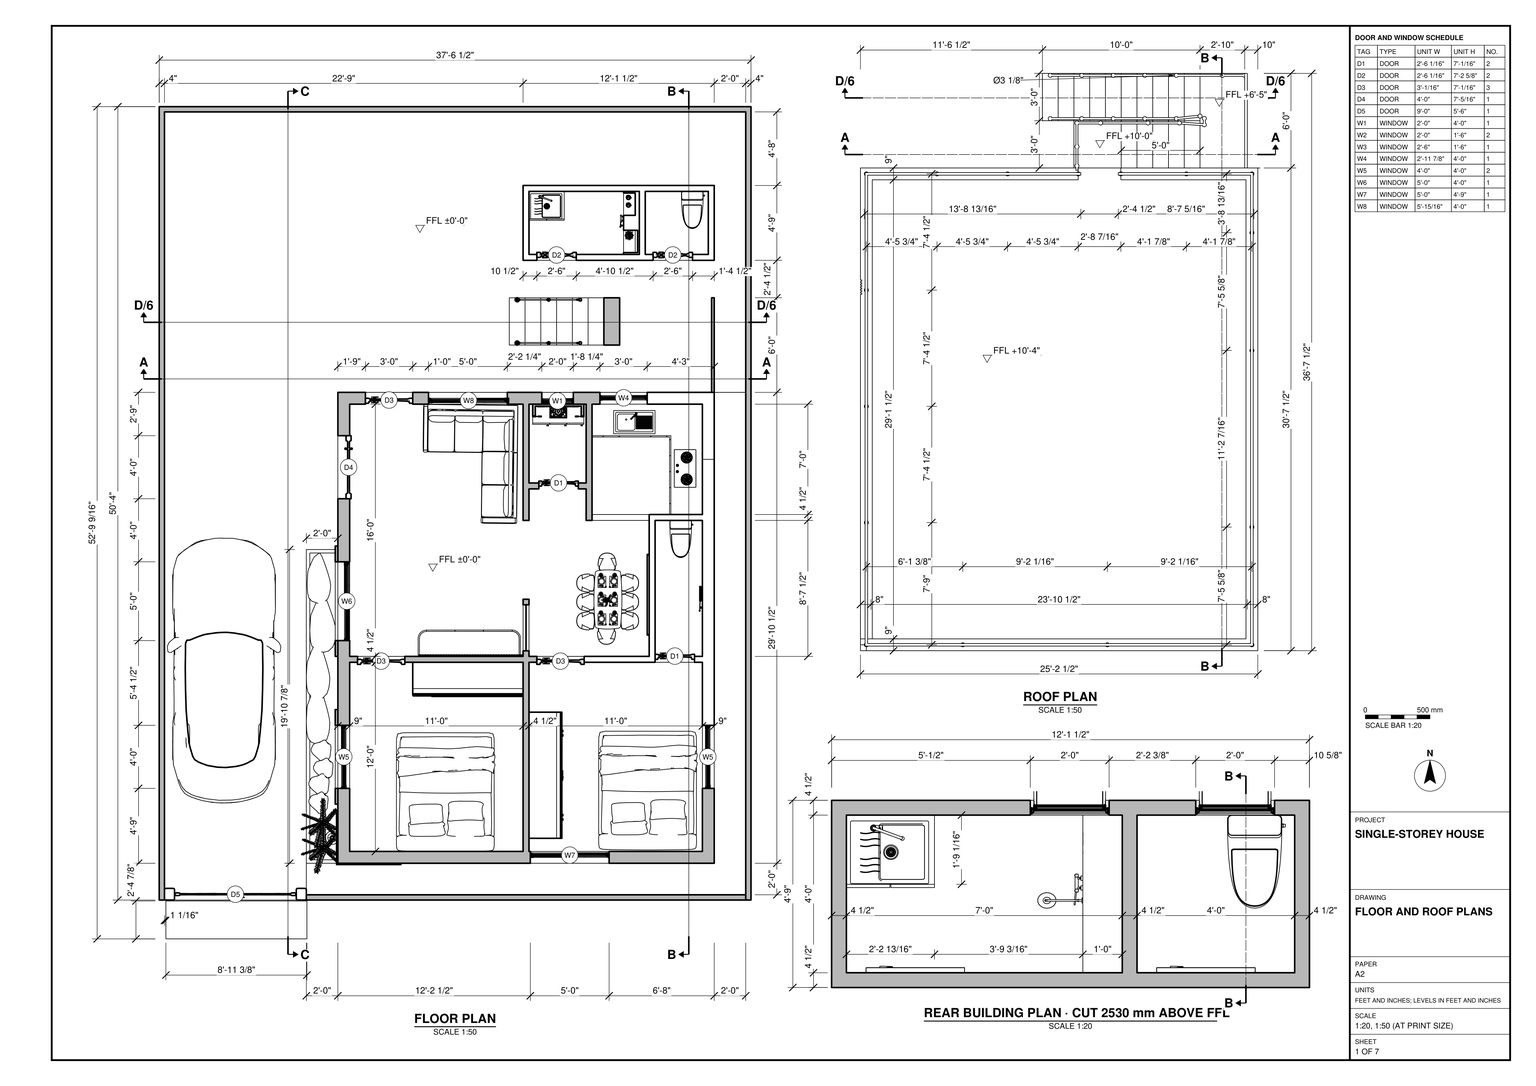
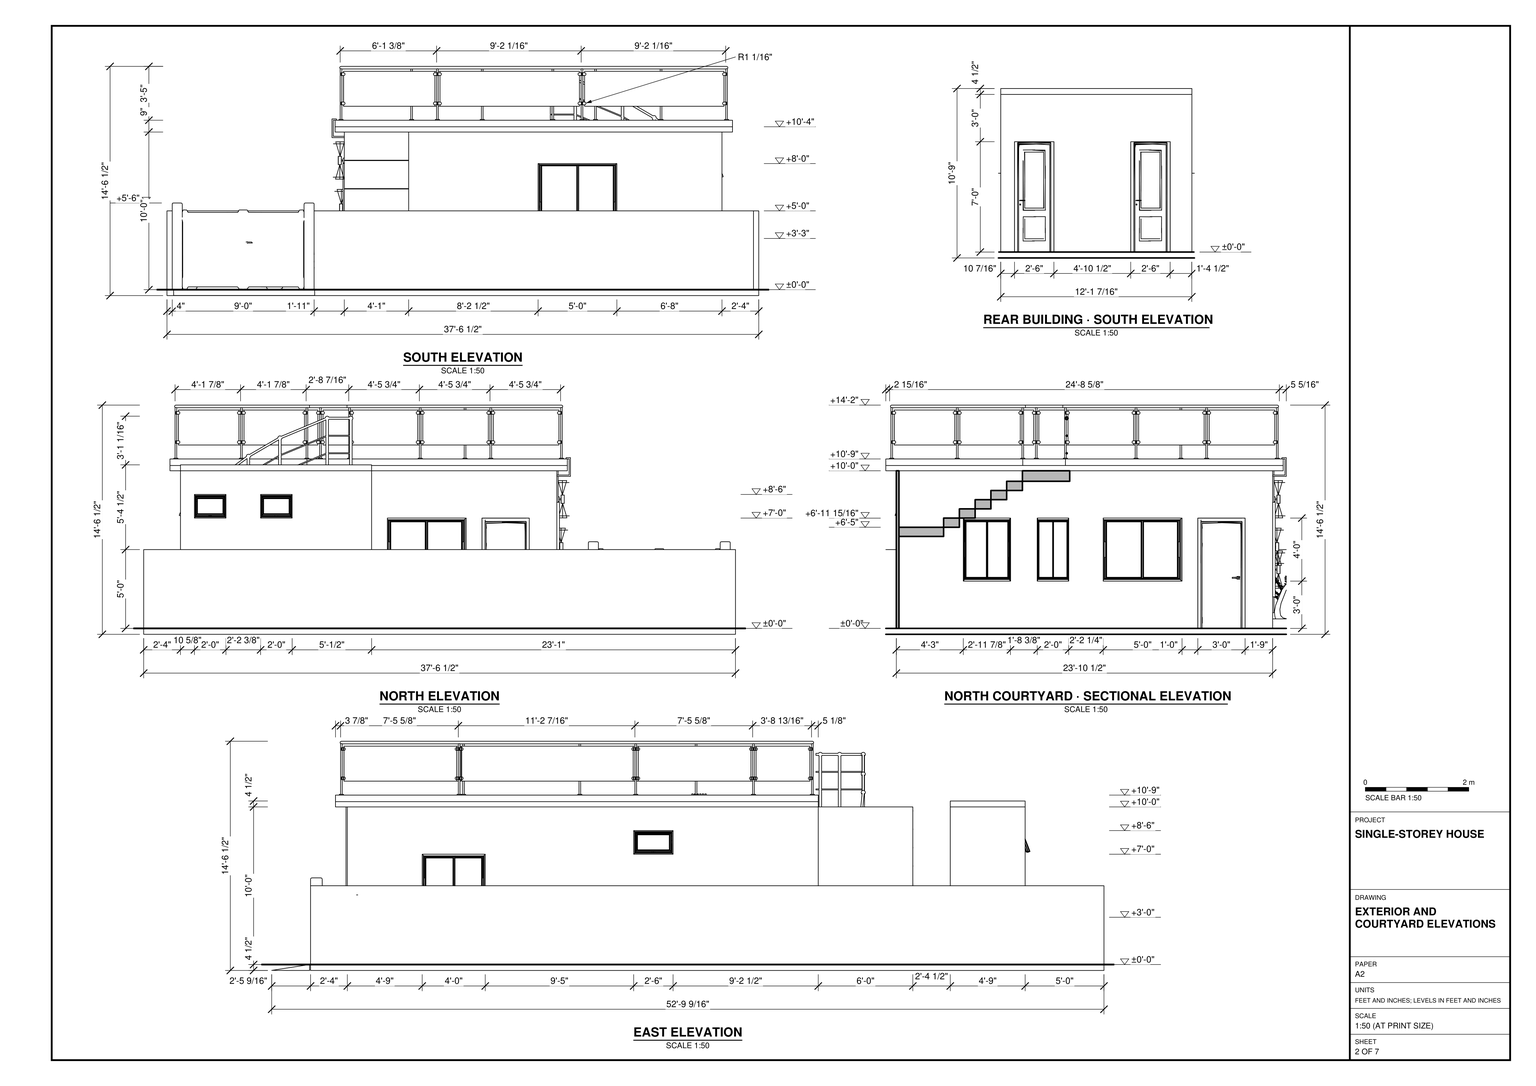
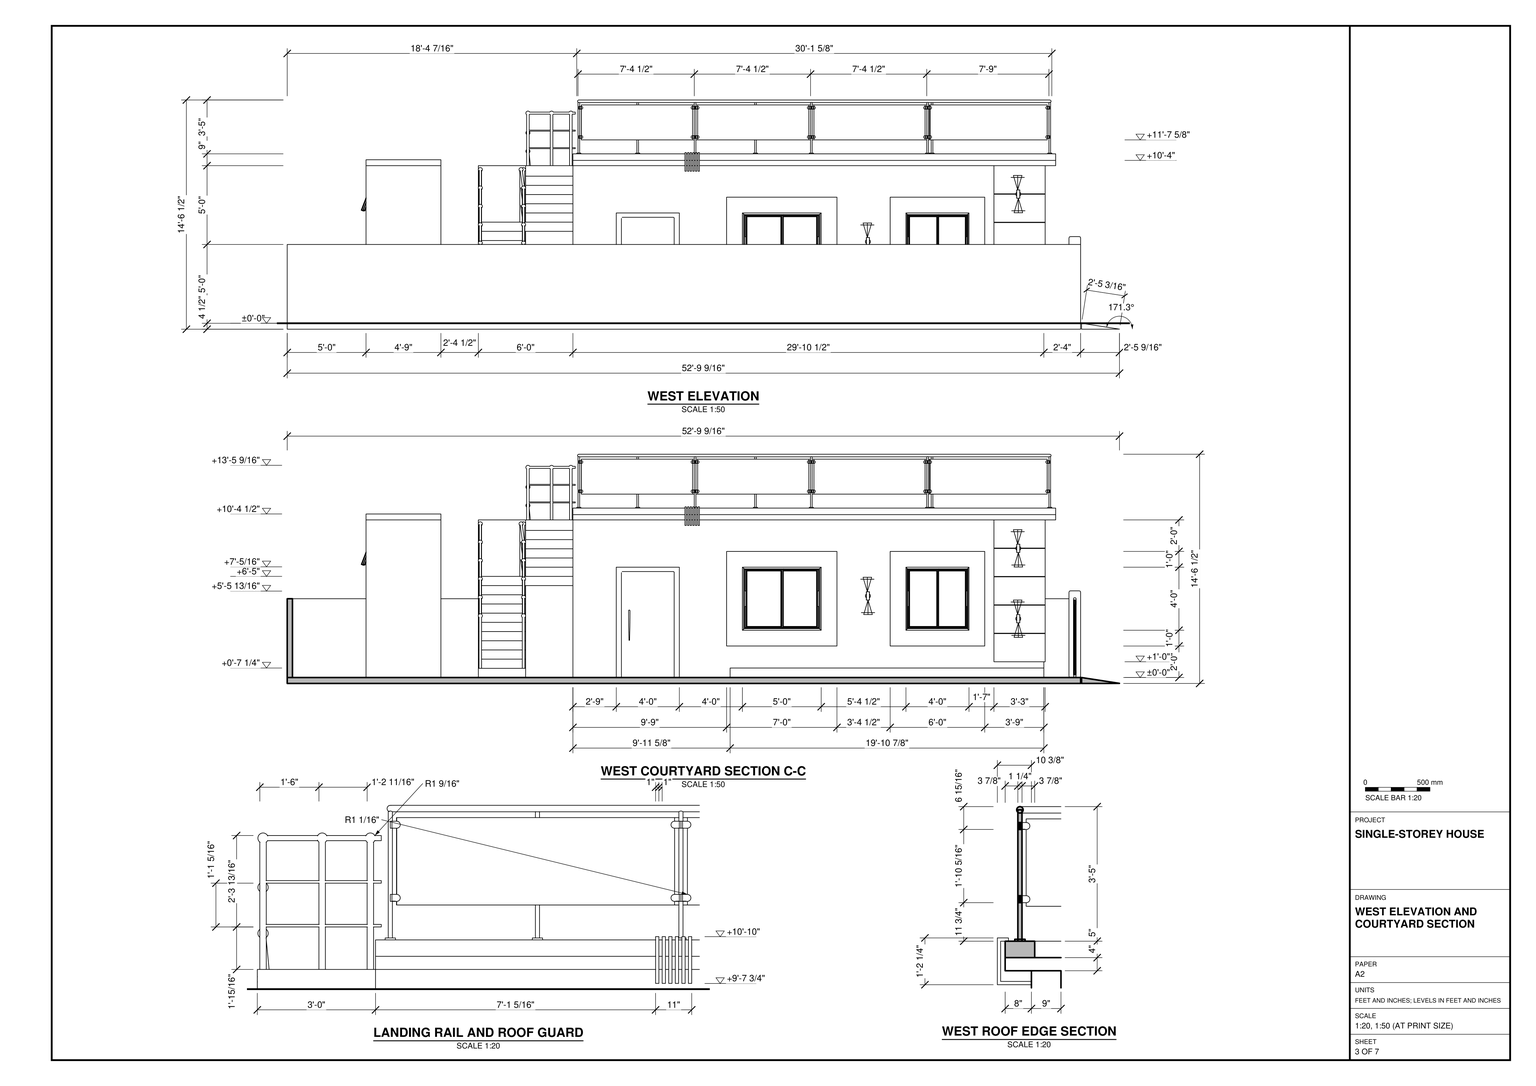
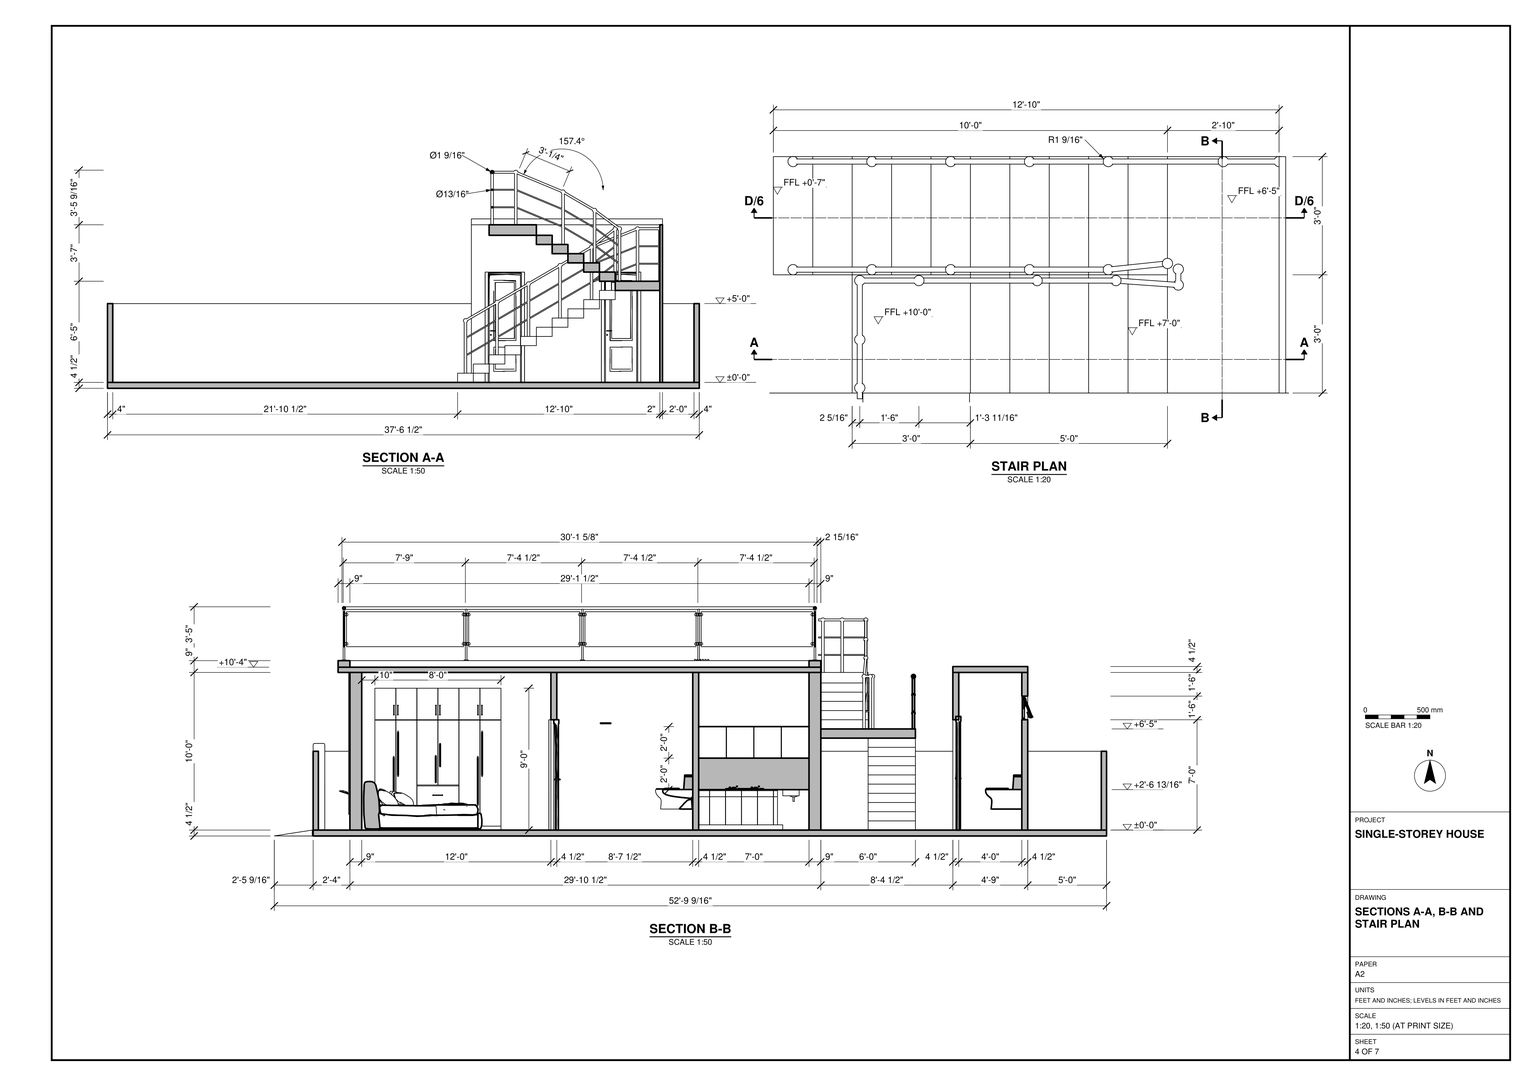
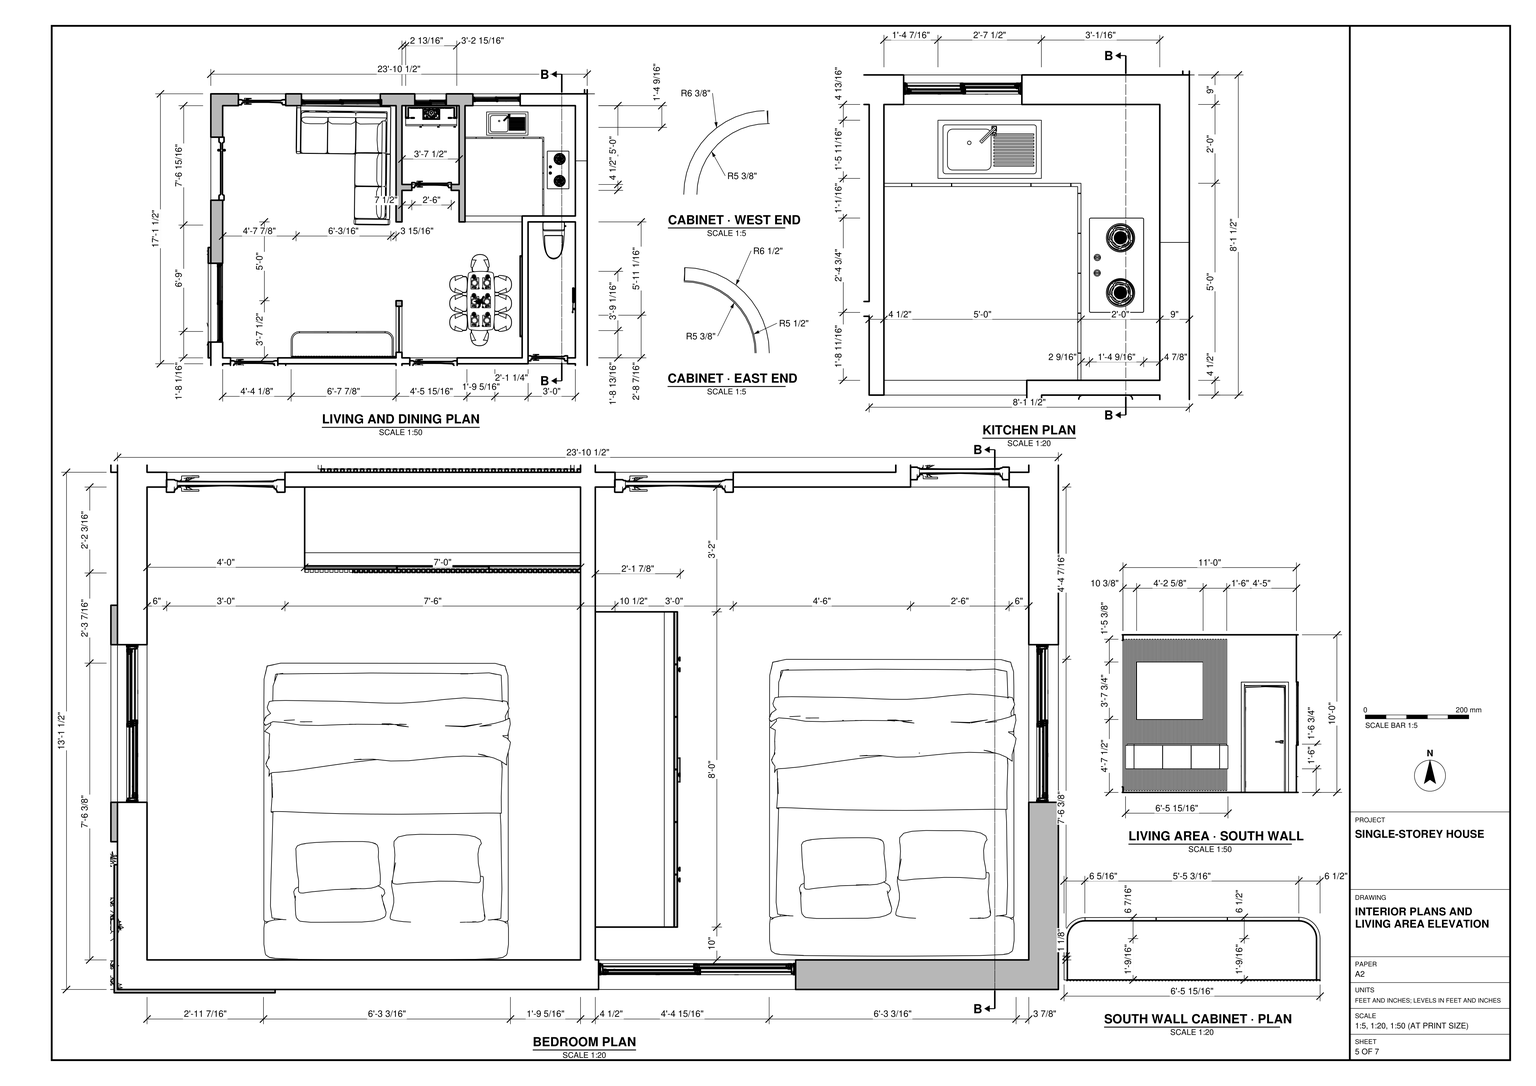
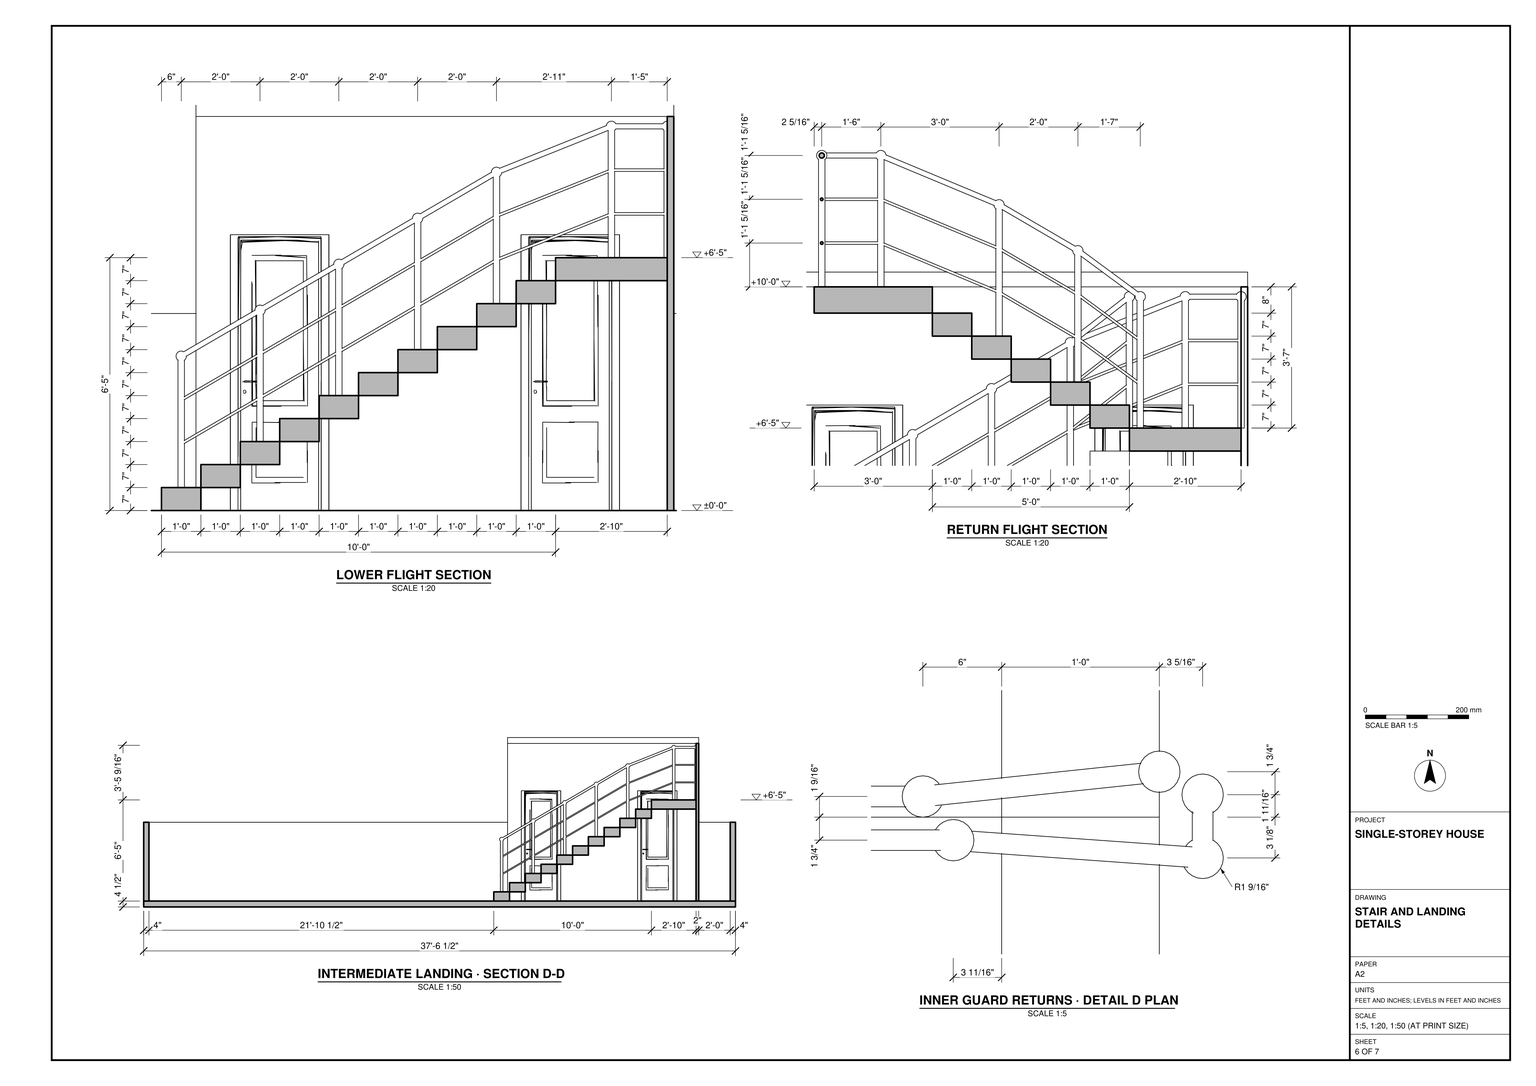
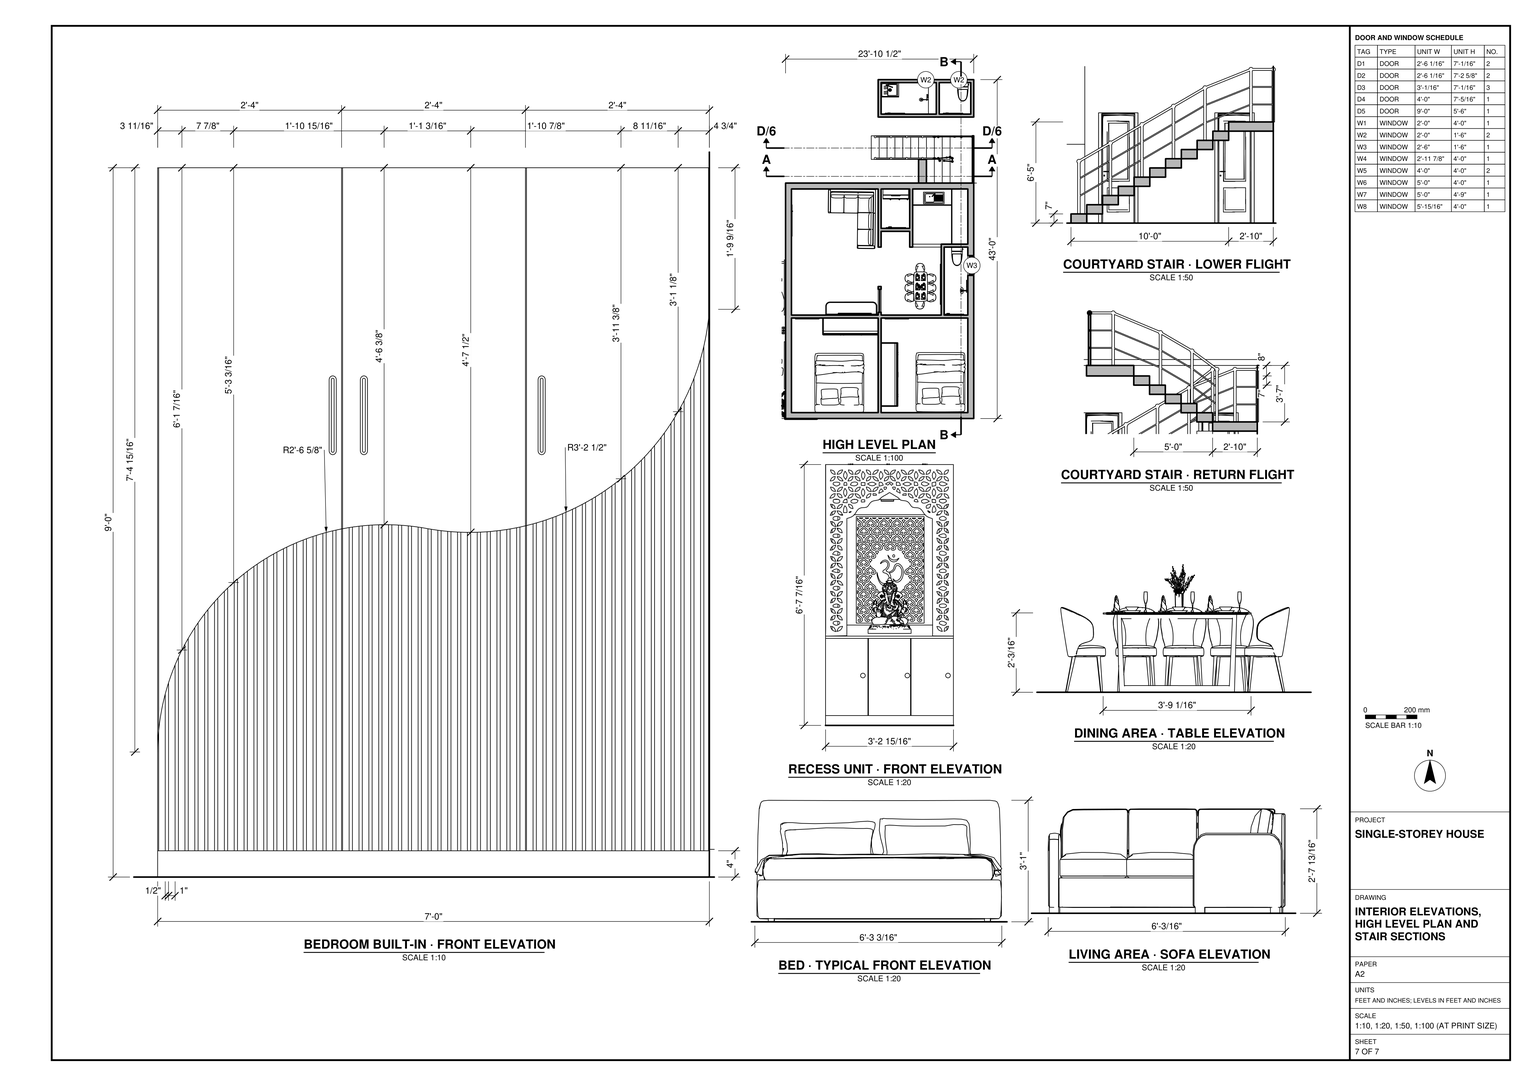
Build the house and its enclosed site in SketchUp using task_files/diagram_01.pdf. Work in feet and inches. Set the ground-floor finished level to ±0'-0". The complete model, including the gate approach and roof guard, measures 37'-6 1/2" east to west, 52'-9 9/16" north to south and 14'-6 1/2" in overall height.

Model the site slab, perimeter walls, vehicle gate and sloped approach. Leave the parking strip west of the house and the courtyard between the house and the detached rear building. Follow the wall thicknesses on the plans, including the 9" main exterior walls and 4 1/2" internal partitions. Form the door and window openings and fit the units according to the schedule and elevations.

Place the two bedrooms along the south side. Follow the plan for the living and dining areas, kitchen counters, plumbing fixtures, beds, sectional sofa, dining table and chairs. Include the car in the parking strip. Give the rear building its separate sink and toilet rooms. Model the exterior stair from the courtyard to the flat roof terrace, including the intermediate landing, handrails and roof-edge guard.

Keep walls, slabs, roofs and each furniture or joinery piece in separate groups or components. Use components for repeated parts. Decor and loose items may be any suitable library components. Save one SketchUp model as output_files/single_storey_house_with_a_courtyard_and_roof_terrace.skp.

# SketchUp Ruby script. Lengths in inches.
U = 1.inch
M = Sketchup.active_model
def pt(a) = Geom::Point3d.new(a.map { |v| v * U })
def face(e, loops, mat)
  f = e.add_face(loops[0].map { |a| pt(a) })
  loops[1..].each { |l| e.add_face(l.map { |a| pt(a) }).erase! }
  f.material = f.back_material = mat if mat
  f
end
# faces: each face lists its corners as indices into pts; further lists are holes
def faces(e, pts, list, mat = nil) = list.each { |f| face(e, (f[0].is_a?(Array) ? f : [f]).map { |l| l.map { |i| pts[i] } }, mat) }
# xy, xz, yz: faces in a plane at the given z, y or x. An outline is a flat list of corners, or four numbers for a rectangle; further outlines are holes
def ring(l) = l.size == 4 ? [[l[0], l[1]], [l[2], l[1]], [l[2], l[3]], [l[0], l[3]]] : l.each_slice(2).to_a
def flat(e, list, mat, &to3) = list.each { |f| face(e, (f[0].is_a?(Array) ? f : [f]).map { |l| ring(l).map { |u, v| to3.(u, v) } }, mat) }
def xy(e, z, list, mat = nil) = flat(e, list, mat) { |x, y| [x, y, z] }
def xz(e, y, list, mat = nil) = flat(e, list, mat) { |x, z| [x, y, z] }
def yz(e, x, list, mat = nil) = flat(e, list, mat) { |y, z| [x, y, z] }
def lines(e, pts, list) = list.each { |a, b| e.add_line(pt(pts[a]), pt(pts[b])) }
# prism: a flat outline (further loops are holes) pulled along v
def prism(e, loops, v, mat = nil)
  f = face(e, loops, mat); d = Geom::Vector3d.new(v.map { |x| x * U })
  f.pushpull(f.normal.samedirection?(d) ? d.length : -d.length)
end
def box(e, o, s, mat = nil) = prism(e, [[o, [o[0] + s[0], o[1], o[2]], [o[0] + s[0], o[1] + s[1], o[2]], [o[0], o[1] + s[1], o[2]]]], [0, 0, s[2]], mat)
def at(x, y, z, deg = 0) = Geom::Transformation.translation(pt([x, y, z])) * Geom::Transformation.rotation(ORIGIN, Z_AXIS, deg.degrees)
def axes(o, x, y, z) = Geom::Transformation.new([*x, 0, *y, 0, *z, 0, *pt(o).to_a, 1])
def part(name) = M.definitions.add(name)
# library, detail: a bought-in or finely detailed component or shape, given as its bounding box
def library(name, o, s) = part(name).tap { |d| box(d.entities, o, s) }
def detail(e, o, s) = box(e.add_group.entities, o, s)
def put(e, d, t, mat = nil) = e.add_instance(d, t).tap { |i| i.material = mat if mat }
def group(e, t, mat = nil) = e.add_group.tap { |g| g.transformation = t; g.material = mat if mat }.entities
root = M.entities
M.materials.add("Bricks A03 100cm").color = [95, 90, 86]
M.materials.add("Carpaint Beige 1.5cm").color = [255, 255, 255]
M.materials.add("Concrete Floor Satin 300cm\#1").color = [133, 133, 131]
M.materials.add("Generic\#2").color = [205, 175, 182]
M.materials["Generic\#2"].alpha = 0.1
M.materials.add("Manhattan Creative Coating MD 1125B 26.44cm\#1").color = [255, 255, 255]
M.materials.add("Sand Stones 01 100cm").color = [188, 164, 143]
M.materials.add("T8500 Silicone plaster D1 27.81cm").color = [255, 255, 255]
M.materials.add("Tiles B 130cm").color = [122, 119, 118]
M.materials.add("Tiles L02 200cm").color = [152, 144, 134]
M.materials.add("Wall Paint Black Satin 300cm").color = [38, 38, 38]
M.materials.add("[Granite Dark Gray]").color = [69, 68, 68]
c1 = library("Archie Sectional",[-59.99,-44.69,0],[94.95,99.96,31.82])
c2 = library("Bed 001",[-37.84,-46.07,0],[75.19,90.39,37.01])
c3 = library("Dining Table",[-4.14,-4.14,0],[95.74,137.21,49.0625])
c4 = library("Print Art 005",[-19,-1,-19.5],[38,1,39])
c5 = library("Window Crafter Awning",[0,-6.05,0],[30,8.26,18])
c6 = library("Toilet\#2",[0.14,-3.79,0],[17.67,28.34,25.87])
c7 = part("Component\#4")
box(c7.entities,[0,-0.25,0],[8.875,17,1])
c8 = library("Shower Raindance Connect",[1.71,-11.67,0],[20.76,23.22,49.85])
c9 = library("Bath Accessories 001",[-1.85,-1.88,0.02],[4.13,3.76,6.42])
c10 = library("Potted Plant 50-23",[-3.4,-3.5,0],[6.8,7,9.93])
c11 = library("items+DOVE",[0,-0.11,-0.26],[16.92,2.54,8.78])
c12 = library("babyshka-cosm",[-31.16,-2.74,2.76],[21.84,5.48,16.53])
c13 = library("skp31A6",[-6.04,-1.48,32.125],[7.16,7.43,5.2])
c14 = library("sink",[0,0,0],[23.82,19.09,24.47])
c15 = library("Door 243 074",[-20.11,-2.41,0],[40.22,4.82,86.63])
c16 = library("Window Crafter Sliding",[0,-0.55,0],[48,4.49,48])
c17 = library("Door 243 053",[-21.6,-2.79,-0.07],[43.2,5.58,82.64])
c18 = library("Door 243 065",[-19.36,-2.49,0],[38.72,4.98,81.96])
c19 = library("Window Crafter Sliding 3",[0,-0.55,0],[60,4.49,93])
c20 = library("Comptonia peregrina 005",[-33.17,-28.03,-1.38],[76.14,61.63,51.11])
c21 = library("Fouquieria splendens 002",[-30.26,-26.69,-2.27],[57.52,65.08,116.59])
c22 = library("Potted Plant 02",[-16.98,-19.78,0],[30.04,38.68,37.52])
c23 = library("Gate 243 002",[-65.73,-4.44,-0.27],[131.46,8.88,65.99])
c24 = library("Car 033",[-43.24,-98.19,-1.29],[86.48,201.64,57.79])
c25 = part("Group1067\#1")
p = [[0,0,0],[0,0,-49.65],[-0.08,0,-49.65],[0.5,-160.25,0],[-0.5,-160.25,0],[0.5,160.25,0],
  [0.5,0,0],[-0.5,160.25,0],[0.08,0,-49.65],[-0.5,0,0],[0,0,-80.375]]
lines(c25.entities,p,[[0,1],[1,2],[3,4],[5,6],[7,5],[1,8],[9,0],[0,6],[8,10],[4,9],[6,3],[2,10],
  [9,7]])
c26 = part("Rectangle Light")
put(c26.entities,c25,at(0,0,0))
c27 = part("Stair flight")
xy(c27.entities,0,[[0,0,12,36]])
xy(c27.entities,7,[[0,0,12,36],[12,0,24,36]])
xy(c27.entities,14,[[12,0,24,36],[24,0,36,36]])
xy(c27.entities,21,[[24,0,36,36],[36,0,48,36]])
xy(c27.entities,28,[[36,0,48,36],[48,0,60,36]])
xy(c27.entities,35,[[48,0,60,36],[60,0,72,36]])
xy(c27.entities,42,[[60,0,72,36],[72,0,84,36]])
xy(c27.entities,49,[[72,0,84,36],[84,0,96,36]])
xy(c27.entities,56,[[84,0,96,36],[96,0,108,36]])
xy(c27.entities,63,[[96,0,108,36],[108,0,120,36]])
xy(c27.entities,70,[[120,-36,154,36],[108,0,120,36]])
xy(c27.entities,77,[[120,-36,154,36]])
xz(c27.entities,-36,[[120,70,154,77]])
xz(c27.entities,0,[[0,0,12,7],[12,7,24,14],[24,14,36,21],[36,21,48,28],[48,28,60,35],
  [60,35,72,42],[72,42,84,49],[84,49,96,56],[96,56,108,63],[108,63,120,70]])
xz(c27.entities,36,[[0,0,12,7],[12,7,24,14],[24,14,36,21],[36,21,48,28],[48,28,60,35],
  [60,35,72,42],[72,42,84,49],[84,49,96,56],[96,56,108,63],[108,63,120,70],
  [120,70,154,77]])
yz(c27.entities,0,[[0,0,36,7]])
yz(c27.entities,12,[[0,0,36,7],[0,7,36,14]])
yz(c27.entities,24,[[0,7,36,14],[0,14,36,21]])
yz(c27.entities,36,[[0,14,36,21],[0,21,36,28]])
yz(c27.entities,48,[[0,21,36,28],[0,28,36,35]])
yz(c27.entities,60,[[0,28,36,35],[0,35,36,42]])
yz(c27.entities,72,[[0,35,36,42],[0,42,36,49]])
yz(c27.entities,84,[[0,42,36,49],[0,49,36,56]])
yz(c27.entities,96,[[0,49,36,56],[0,56,36,63]])
yz(c27.entities,108,[[0,56,36,63],[0,63,36,70]])
yz(c27.entities,120,[[0,63,36,70],[-36,70,36,77]])
yz(c27.entities,154,[[-36,70,36,77]])
c28 = part("Group\#4")
box(c28.entities,[0,0,0],[12,36,7])
c29 = library("Group\#12",[0,0,0],[151.15,73.82,154.57])
c30 = library("Group\#40",[0,0,0],[38.9375,16.5625,79.4375])
c31 = library("Group\#43",[0,0,0],[25.875,96,108])
c32 = library("Group\#51",[0,0,0],[84,26.16,108])
c33 = library("Group\#52",[0,0,0],[84,84,78.79])
c34 = library("Group\#53",[0,0,0],[79.9,20.09,115.27])
c35 = library("Group\#55",[0,0,0],[24.8,71.0625,68])
c36 = library("Group\#57",[0,0,0],[296.65,361.65,40.98])
c37 = part("Group\#21")
prism(c37.entities,[[[0,1,14.25],[3.375,1,14.25],[3.375,1,13.25],[1,1,13.25],[1,1,1],[10.375,1,1],[10.375,1,0],[0,1,0]]],[0,-1,0])
c38 = library("Group\#62",[0,0,0],[10.39,10.72,28.4])
box(root,[420.5,416.07,4.5],[2,72,120])
box(root,[282.5,57.57,4.5],[60,9,39])
xy(root,124.5,[[128,372.98,129,373.98]])
yz(root,353.5,[[550.82,5.75,567.82,21.85],[522.47,5.9,539.47,21.99]])
p = [[278.5,488.07,4.5],[278.5,452.07,4.5],[277,215.07,121.125],[277,215.07,4.5],[541.11,65.54,57.51],[541.11,64.54,57.51],
  [293.76,411.57,133.5],[240.01,411.57,133.5],[132.5,411.57,133.5],[132.5,323.07,133.5],[137,57.57,133.5],[128,57.57,133.5],
  [132.5,53.07,133.5],[132.5,48.57,133.5],[128,53.07,133.5],[426,411.57,133.5],[326.23,411.57,133.5],[186.25,411.57,133.5],
  [132.5,234.57,133.5],[132.5,146.07,133.5],[426,232.32,133.5],[426,321.95,133.5]]
lines(root,p,[[0,1],[2,3],[4,5],[6,7],[8,9],[10,11],[12,13],[12,14],[15,16],[7,17],[17,8],[9,18],
  [18,19],[20,21],[21,15]])
put(root,c1,axes([232.77,349.74,4.5],[-0.01015,-0.94995,0],[0.71996,-0.00769,0],[0,0,1]))
put(root,c2,at(217.82,110.89,4.5,180))
put(root,c2,at(371.8,112.04,4.5,180))
put(root,c3,axes([317.76,224.21,4.5],[0.54,0,0],[0,0.54,0],[0,0,0.7938]))
put(root,c4,axes([373,261.98,73.15],[0,-1.6157,0],[1.51,0,0],[0,0,1.1325]))
put(root,c5,at(417.46,275.5625,88.5,90))
put(root,c6,at(397.39,544.52,20.5))
put(root,c7,at(353.5,551.07,21.85))
put(root,c7,at(353.5,522.72,21.99))
put(root,c7,at(353.5,551.07,37.95))
put(root,c7,at(353.5,522.72,38.09))
put(root,c7,at(353.5,551.07,54.05))
put(root,c7,at(353.5,522.72,54.19))
put(root,c7,at(353.5,551.07,70.15))
put(root,c7,at(353.5,522.72,70.29))
put(root,c8,axes([346.66,552.01,34.2],[0,-0.50278,0],[0.59212,0,0],[0,0,1]))
put(root,c9,at(357.18,564.42,38.95))
put(root,c9,at(357.09,534.625,22.99))
put(root,c10,at(358.07,563.71,22.85))
put(root,c10,at(357.82,535.38,39.09))
put(root,c10,at(362.375,525.01,71.29))
put(root,c11,axes([359.39,566.73,55.05],[0,-0.7,0],[0.7,0,0],[0,0,0.7]))
put(root,c12,axes([358.9375,521.62,54],[0,-0.43,0],[0.43,0,0],[0,0,0.43]))
put(root,c13,at(359.54,558.27,39.02))
put(root,c9,at(357.18,558.67,38.95))
put(root,c14,at(282.74,548.21,18.9375))
put(root,c15,axes([390.97,520.66,4.43],[0.7469,0,0],[0,1,0],[0,0,1]))
put(root,c16,at(419.32,114.57,40.5,90))
put(root,c17,axes([144.14,359.07,4.57],[0,1.11105,0],[-1,0,0],[0,0,1.02]))
put(root,c15,axes([302.48,520.66,4.43],[0.7469,0,0],[0,1,0],[0,0,1]))
put(root,c5,axes([411.875,571.28,88.5],[-0.8,0,0],[0,-1,0],[0,0,1]))
put(root,c16,axes([205,408.18,40.5],[1.27,0,0],[0,1,0],[0,0,1]))
put(root,c18,axes([174.96,410.23,4.43],[0.93195,0,0],[0,1,0],[0,0,1.02567]))
put(root,c16,at(142.1875,114.57,40.5,90))
put(root,c18,axes([305.45,211.48,4.43],[0.93195,0,0],[0,1,0],[0,0,1.02567]))
put(root,c16,axes([291.25,407.9,40.5],[0.5,0,0],[0,1,0],[0,0,1]))
put(root,c16,axes([144.4375,227.07,40.5],[0,1.25,0],[-1,0,0],[0,0,1]))
put(root,c19,axes([282.5,62.07,43.5],[1,0,0],[0,1,0],[0,0,0.6129]))
put(root,c18,axes([168.95,211.48,4.43],[0.93195,0,0],[0,1,0],[0,0,1.02567]))
put(root,c18,axes([392.52,215.28,4.45],[0.77578,0,0],[0,1,0],[0,0,1.02567]))
put(root,c16,axes([335.6,410.23,40.5],[0.74786,0,0],[0,1,0],[0,0,1]))
put(root,c18,axes([304.03,347.18,4.5],[0.77578,0,0],[0,1,0],[0,0,1.02567]))
put(root,c5,axes([361.5,571.28,88.5],[-0.8,0,0],[0,-1,0],[0,0,1]))
put(root,c20,axes([120.42,272.81,12.47],[0.23515,0,0],[0,0.624,0],[0,0,0.52214]))
put(root,c20,axes([123.38,237.89,10.24],[0.26337,0,0],[0,0.69888,0],[0,0,0.56489]))
put(root,c20,axes([119.8,202.2,12.47],[0.23515,0,0],[0,0.69548,0],[0,0,0.51795]))
put(root,c20,axes([119.8,168.38,12.46],[0.23515,0,0],[0,0.73316,0],[0,0,0.51596]))
put(root,c21,axes([123.61,141.39,7.78],[0.2622,0,0],[0,0.2622,0],[0,0,0.2622]))
put(root,c21,axes([125.28,127.79,7.77],[0.2584,0,0],[0,0.2584,0],[0,0,0.2584]))
put(root,c21,axes([122.04,115.57,7.8],[0.2679,0,0],[0,0.2679,0],[0,0,0.2679]))
put(root,c21,axes([121.63,102.21,7.76],[0.2546,0,0],[0,0.2546,0],[0,0,0.2546]))
put(root,c22,at(125.01,69.22,7.1875))
put(root,c22,at(124.78,88.36,7.1875))
put(root,c23,axes([58,34.01,4.77],[0.82148,0,0],[0,1,0],[0,0,1]))
put(root,c24,at(49.36,206.93,5.79,180))
put(root,c26,axes([135.5,255.82,124.49],[-1,0,0],[0,-1,0],[0,0,0.0132]))
g1 = group(root,at(0,29.57,0))
xy(g1,0,[[0,0,450.5,604]])
xy(g1,4.5,[[0,0,4,0,4,600,446.5,600,446.5,386.5,136,386.5,136,266.85,112,266.85,112,0,450.5,0,450.5,604,0,604]])
xy(g1,4.5,[[4,0,112,0,112,266.85,136,266.85,136,386.5,446.5,386.5,446.5,600,4,600]],"Tiles B 130cm")
xz(g1,0,[[0,0,450.5,4.5]])
xz(g1,604,[[0,0,450.5,4.5]])
yz(g1,0,[[0,0,604,4.5]])
yz(g1,450.5,[[0,0,604,4.5]])
g2 = group(root,at(136,57.57,124.5))
xy(g2,0,[[-8,-9,294.5,358.5]])
xy(g2,4,[[-8,-9,294.5,358.5]],"Concrete Floor Satin 300cm\#1")
xz(g2,-9,[[-8,0,294.5,4]],"Wall Paint Black Satin 300cm")
xz(g2,358.5,[[-8,0,294.5,4]],"Wall Paint Black Satin 300cm")
yz(g2,-8,[[-9,0,358.5,4]],"Wall Paint Black Satin 300cm")
yz(g2,294.5,[[-9,0,358.5,4]],"Wall Paint Black Satin 300cm")
g3 = group(root,at(277,516.57,4.5),"Carpaint Beige 1.5cm")
xy(g3,0,[[0,0,0,57,145.5,57,145.5,0,129,0,129,4.5,141,4.5,141,52.5,93,52.5,93,4.5,99,4.5,99,0,40.5,0,40.5,4.5,88.5,4.5,88.5,52.5,4.5,52.5,4.5,4.5,10.5,4.5,10.5,0],[10.5,0,40.5,0,40.5,4.5,88.5,4.5,88.5,52.5,4.5,52.5,4.5,4.5,10.5,4.5],[99,0,129,0,129,4.5,141,4.5,141,52.5,93,52.5,93,4.5,99,4.5]])
xy(g3,84,[[10.5,0,40.5,4.5],[99,0,129,4.5],[60.5,52.5,84.5,57],[110.875,52.5,134.875,57]])
xy(g3,102,[[60.5,52.5,84.5,57],[110.875,52.5,134.875,57]])
xy(g3,120,[[[0,0,145.5,57],[4.5,4.5,88.5,52.5],[93,4.5,141,52.5]]])
xz(g3,0,[[0,0,10.5,0,10.5,84,40.5,84,40.5,0,99,0,99,84,129,84,129,0,145.5,0,145.5,120,0,120]])
xz(g3,4.5,[[4.5,0,4.5,120,88.5,120,88.5,0,40.5,0,40.5,84,10.5,84,10.5,0],[93,0,93,120,141,120,141,0,129,0,129,84,99,84,99,0]])
xz(g3,52.5,[[[4.5,0,88.5,120],[60.5,84,84.5,102]],[[93,0,141,120],[110.875,84,134.875,102]]])
xz(g3,57,[[[0,0,145.5,120],[60.5,84,84.5,102],[110.875,84,134.875,102]]])
yz(g3,0,[[0,0,57,120]])
yz(g3,4.5,[[4.5,0,52.5,120]])
yz(g3,10.5,[[0,0,4.5,84]])
yz(g3,40.5,[[0,0,4.5,84]])
yz(g3,60.5,[[52.5,84,57,102]])
yz(g3,84.5,[[52.5,84,57,102]])
yz(g3,88.5,[[4.5,0,52.5,120]])
yz(g3,93,[[4.5,0,52.5,120]])
yz(g3,99,[[0,0,4.5,84]])
yz(g3,110.875,[[52.5,84,57,102]])
yz(g3,129,[[0,0,4.5,84]])
yz(g3,134.875,[[52.5,84,57,102]])
yz(g3,141,[[4.5,0,52.5,120]])
yz(g3,145.5,[[0,0,57,120]])
g4 = group(root,at(266.5,416.07,4.5),"Tiles L02 200cm")
put(g4,c27,at(0,36,0))
put(g4,c28,at(108,0,77))
put(g4,c28,at(84,0,91))
put(g4,c28,at(72,0,98))
g5 = group(g4,at(48,0,112))
box(g5,[-24,0,0],[36,36,8])
put(g4,c28,at(96,0,84))
put(g4,c28,at(60,0,105))
put(root,c29,at(270.93,414.32,11.5))
g6 = group(root,at(329.5,323.07,4.5))
xy(g6,4,[[60,0,64,64],[0,60,60,64]],"[Granite Dark Gray]")
xz(g6,60,[[0,4,60,25.38]],"[Granite Dark Gray]")
xz(g6,64,[[0,0,64,4]],"[Granite Dark Gray]")
yz(g6,60,[[0,4,60,25.38]],"[Granite Dark Gray]")
yz(g6,64,[[0,0,64,4]],"[Granite Dark Gray]")
p = [[84,0,0],[64,0,0],[84,84,0],[0,84,0],[0,64,0]]
lines(g6,p,[[0,1],[2,3],[3,4]])
put(root,c30,at(284.32,390.51,4.5))
put(root,c31,at(281.5,76.57,4.5))
g7 = group(root,at(353.5,521.07,4.5))
xy(g7,0,[[0,0,12,48]])
xy(g7,1.25,[[0,29.75,8.875,46.75]])
xy(g7,1.4,[[0,1.4,10.6875,18.4]])
xy(g7,82.6,[[0,1.4,10.6875,18.4]])
xy(g7,82.75,[[0,29.75,8.875,46.75]])
xy(g7,84,[[0,0,12,48]])
xz(g7,0,[[0,0,12,84]])
xz(g7,1.4,[[0,1.4,10.6875,82.6]])
xz(g7,18.4,[[0,1.4,10.6875,82.6]])
xz(g7,29.75,[[0,1.25,8.875,82.75]])
xz(g7,46.75,[[0,1.25,8.875,82.75]])
xz(g7,48,[[0,0,12,84]])
yz(g7,0,[[0,0,0,84,18,84,18,82.6,1.4,82.6,1.4,1.4,18,1.4,18,0],[18,0,18,1.4,18.4,1.4,18.4,82.6,18,82.6,18,84,30,84,30,82.75,29.75,82.75,29.75,1.25,46.75,1.25,46.75,82.75,30,82.75,30,84,48,84,48,0]])
yz(g7,8.875,[[29.75,1.25,46.75,82.75]])
yz(g7,10.6875,[[1.4,1.4,18.4,82.6]])
yz(g7,12,[[0,0,48,84]])
g8 = group(root,at(281.5,554.57,4.5))
p = [[10.286,3.208,24],[10.287,3.087,24],[10.281,2.959,24],[10.282,2.959,24],[10.282,3.265,24]]
lines(g8,p,[[0,1],[2,3],[4,0]])
detail(g8,[0,-6.5625,0],[26.8125,21.0625,24])
g9 = group(root,at(281.5,547.01,6.3125))
xy(g9,0,[[0,0,13.25,1],[13.5625,0,26.8125,1]])
xy(g9,22.1875,[[0,0,13.25,1],[13.5625,0,26.8125,1]])
xz(g9,0,[[0,0,13.25,22.1875],[13.5625,0,26.8125,22.1875]])
xz(g9,1,[[0,0,13.25,22.1875],[13.25,0,13.5625,22.1875],[13.5625,0,26.8125,22.1875]])
yz(g9,0,[[0,0,1,22.1875]])
yz(g9,13.25,[[0,0,1,22.1875]])
yz(g9,13.5625,[[0,0,1,22.1875]])
yz(g9,26.8125,[[0,0,1,22.1875]])
g10 = group(root,at(277,516.57,124.5),"Manhattan Creative Coating MD 1125B 26.44cm\#1")
box(g10,[0,0,0],[145.5,57,4.5])
g11 = group(root,at(0,29.57,4.5),"T8500 Silicone plaster D1 27.81cm")
prism(g11,[[[0,604,0],[450.5,604,0],[450.5,0,0],[446.5,0,0],[446.5,600,0],[4,600,0],[4,0,0],[0,0,0]]],[0,0,60])
put(root,c32,at(193,184.41,4.5))
put(root,c33,at(329.5,323.07,4.5))
put(root,c34,at(197.1,215.07,5.85))
put(root,c35,at(388.7,247.51,20.5))
g12 = group(root,at(128,48.57,128.5),"Wall Paint Black Satin 300cm")
prism(g12,[[[293.5,358.5,0],[198.23,358.5,0],[198.23,367.5,0],[302.5,367.5,0],[302.5,0,0],[0,0,0],[0,367.5,0],[165.76,367.5,0],[165.76,358.5,0],[9,358.5,0],[9,9,0],[293.5,9,0]]],[0,0,5])
put(root,c36,at(130.93,51.5,133.5))
g13 = group(root,at(136,57.57,4.5))
yz(g13,143.25,[[161.72,4.22,196.78,115.78]],"Generic\#2")
g14 = group(g13,at(0,0,0))
xy(g14,0,[[0,0,0,277.5,9,277.5,9,157.5,15,157.5,15,153,9,153,9,9,141,9,141,153,51,153,51,157.5,141,157.5,141,201,145.5,201,145.5,157.5,151.5,157.5,151.5,153,145.5,153,145.5,9,146.5,9,146.5,0],[146.5,0,206.5,0,206.5,9,277.5,9,277.5,153,187.5,153,187.5,157.5,151.5,157.5,151.5,153,145.5,153,145.5,9,146.5,9],[206.5,0,206.5,9,277.5,9,277.5,153,271.5,153,271.5,157.5,277.5,157.5,277.5,261,241.5,261,241.5,153,187.5,153,187.5,157.5,237,157.5,237,265.5,277.5,265.5,277.5,307.5,286.5,307.5,286.5,0],[9,9,141,9,141,153,51,153,51,157.5,15,157.5,15,153,9,153],[241.5,153,271.5,153,271.5,157.5,277.5,157.5,277.5,261,241.5,261],
  [9,157.5,141,157.5,141,201,145.5,201,145.5,157.5,237,157.5,237,261,189,261,189,285,183,285,183,289.5,153,289.5,153,285,145.5,285,145.5,261,141,261,141,349.5,57,349.5,57,358.5,21,358.5,21,349.5,9,349.5,9,325.5,0,325.5,0,277.5,9,277.5],[141,261,141,349.5,57,349.5,57,358.5,286.5,358.5,286.5,307.5,277.5,307.5,277.5,349.5,193.5,349.5,193.5,261,189,261,189,285,183,285,183,289.5,189,289.5,189,349.5,145.5,349.5,145.5,289.5,153,289.5,153,285,145.5,285,145.5,261],[193.5,261,237,265.5],[193.5,265.5,277.5,349.5],[145.5,289.5,189,349.5],
  [0,325.5,0,358.5,21,358.5,21,349.5,9,349.5,9,325.5]],"Carpaint Beige 1.5cm")
xy(g14,4.22,[[141,161.72,145.5,196.78]],"Carpaint Beige 1.5cm")
xy(g14,36,[[0,57,9,105],[277.5,57,286.5,105],[0,169.5,9,229.5],[69,349.5,129,358.5],[155.25,349.5,179.25,358.5],
  [199.5,349.5,235.5,358.5]],"Carpaint Beige 1.5cm")
xy(g14,84,[[0,57,9,105],[277.5,57,286.5,105],[15,153,51,157.5],[151.5,153,187.5,157.5],[241.5,153,271.5,157.5],
  [0,169.5,9,229.5],[277.5,217.99,286.5,247.99],[0,277.5,9,325.5],[153,285,183,289.5],[21,349.5,57,358.5],
  [69,349.5,129,358.5],[155.25,349.5,179.25,358.5],[199.5,349.5,235.5,358.5]],"Carpaint Beige 1.5cm")
xy(g14,96,[[146.5,0,206.5,9]],"Carpaint Beige 1.5cm")
xy(g14,102,[[277.5,217.99,286.5,247.99]],"Carpaint Beige 1.5cm")
xy(g14,115.78,[[141,161.72,145.5,196.78]],"Carpaint Beige 1.5cm")
xy(g14,120,[[[0,0,286.5,358.5],[9,157.5,9,349.5,141,349.5,141,261,145.5,261,145.5,285,189,285,189,261,193.5,261,193.5,349.5,277.5,349.5,277.5,265.5,237,265.5,237,157.5,145.5,157.5,145.5,201,141,201,141,157.5],[145.5,9,277.5,153],[9,9,141,153],[241.5,157.5,277.5,261],[145.5,289.5,189,349.5]]],"Carpaint Beige 1.5cm")
xz(g14,0,[[0,0,146.5,0,146.5,96,206.5,96,206.5,0,286.5,0,286.5,120,0,120]],"Carpaint Beige 1.5cm")
xz(g14,9,[[9,0,141,120],[145.5,0,145.5,120,277.5,120,277.5,0,206.5,0,206.5,96,146.5,96,146.5,0]],"Carpaint Beige 1.5cm")
xz(g14,57,[[0,36,9,84],[277.5,36,286.5,84]],"Carpaint Beige 1.5cm")
xz(g14,105,[[0,36,9,84],[277.5,36,286.5,84]],"Carpaint Beige 1.5cm")
xz(g14,153,[[9,0,15,0,15,84,51,84,51,0,141,0,141,120,9,120],[145.5,0,151.5,0,151.5,84,187.5,84,187.5,0,241.5,0,241.5,84,271.5,84,271.5,0,277.5,0,277.5,120,145.5,120]],"Carpaint Beige 1.5cm")
xz(g14,157.5,[[9,0,9,120,141,120,141,0,51,0,51,84,15,84,15,0],[145.5,0,145.5,120,237,120,237,0,187.5,0,187.5,84,151.5,84,151.5,0],[271.5,0,271.5,84,241.5,84,241.5,120,277.5,120,277.5,0]],"Carpaint Beige 1.5cm")
xz(g14,161.72,[[141,4.22,145.5,115.78]],"Carpaint Beige 1.5cm")
xz(g14,169.5,[[0,36,9,84]],"Carpaint Beige 1.5cm")
xz(g14,196.78,[[141,4.22,145.5,115.78]],"Carpaint Beige 1.5cm")
xz(g14,201,[[141,0,145.5,120]],"Carpaint Beige 1.5cm")
xz(g14,217.99,[[277.5,84,286.5,102]],"Carpaint Beige 1.5cm")
xz(g14,229.5,[[0,36,9,84]],"Carpaint Beige 1.5cm")
xz(g14,247.99,[[277.5,84,286.5,102]],"Carpaint Beige 1.5cm")
xz(g14,261,[[141,0,145.5,120],[189,0,193.5,120],[241.5,0,277.5,120]],"Carpaint Beige 1.5cm")
xz(g14,265.5,[[237,0,277.5,120]],"Carpaint Beige 1.5cm")
xz(g14,277.5,[[0,0,9,84]],"Carpaint Beige 1.5cm")
xz(g14,285,[[145.5,0,153,0,153,84,183,84,183,0,189,0,189,120,145.5,120]],"Carpaint Beige 1.5cm")
xz(g14,289.5,[[145.5,0,145.5,120,189,120,189,0,183,0,183,84,153,84,153,0]],"Carpaint Beige 1.5cm")
xz(g14,325.5,[[0,0,9,84]],"Carpaint Beige 1.5cm")
xz(g14,349.5,[[[9,0,21,0,21,84,57,84,57,0,141,0,141,120,9,120],[69,36,129,84]],[[145.5,0,189,120],[155.25,36,179.25,84]],[[193.5,0,277.5,120],[199.5,36,235.5,84]]],"Carpaint Beige 1.5cm")
xz(g14,358.5,[[[0,0,0,120,286.5,120,286.5,0,57,0,57,84,21,84,21,0],[69,36,129,84],[199.5,36,235.5,84],[155.25,36,179.25,84]]],"Carpaint Beige 1.5cm")
yz(g14,0,[[[0,0,0,120,358.5,120,358.5,0,325.5,0,325.5,84,277.5,84,277.5,0],[169.5,36,229.5,84],[57,36,105,84]]],"Carpaint Beige 1.5cm")
yz(g14,9,[[[9,0,153,120],[57,36,105,84]],[[157.5,0,277.5,0,277.5,84,325.5,84,325.5,0,349.5,0,349.5,120,157.5,120],[169.5,36,229.5,84]]],"Carpaint Beige 1.5cm")
yz(g14,15,[[153,0,157.5,84]],"Carpaint Beige 1.5cm")
yz(g14,21,[[349.5,0,358.5,84]],"Carpaint Beige 1.5cm")
yz(g14,51,[[153,0,157.5,84]],"Carpaint Beige 1.5cm")
yz(g14,57,[[349.5,0,358.5,84]],"Carpaint Beige 1.5cm")
yz(g14,69,[[349.5,36,358.5,84]],"Carpaint Beige 1.5cm")
yz(g14,129,[[349.5,36,358.5,84]],"Carpaint Beige 1.5cm")
yz(g14,141,[[9,0,153,120],[[157.5,0,201,120],[161.72,4.22,196.78,115.78]],[261,0,349.5,120]],"Carpaint Beige 1.5cm")
yz(g14,145.5,[[9,0,153,120],[[157.5,0,201,120],[161.72,4.22,196.78,115.78]],[261,0,285,120],[289.5,0,349.5,120]],"Carpaint Beige 1.5cm")
yz(g14,146.5,[[0,0,9,96]],"Carpaint Beige 1.5cm")
yz(g14,151.5,[[153,0,157.5,84]],"Carpaint Beige 1.5cm")
yz(g14,153,[[285,0,289.5,84]],"Carpaint Beige 1.5cm")
yz(g14,155.25,[[349.5,36,358.5,84]],"Carpaint Beige 1.5cm")
yz(g14,179.25,[[349.5,36,358.5,84]],"Carpaint Beige 1.5cm")
yz(g14,183,[[285,0,289.5,84]],"Carpaint Beige 1.5cm")
yz(g14,187.5,[[153,0,157.5,84]],"Carpaint Beige 1.5cm")
yz(g14,189,[[261,0,285,120],[289.5,0,349.5,120]],"Carpaint Beige 1.5cm")
yz(g14,193.5,[[261,0,349.5,120]],"Carpaint Beige 1.5cm")
yz(g14,199.5,[[349.5,36,358.5,84]],"Carpaint Beige 1.5cm")
yz(g14,206.5,[[0,0,9,96]],"Carpaint Beige 1.5cm")
yz(g14,235.5,[[349.5,36,358.5,84]],"Carpaint Beige 1.5cm")
yz(g14,237,[[157.5,0,265.5,120]],"Carpaint Beige 1.5cm")
yz(g14,241.5,[[153,0,261,0,261,120,157.5,120,157.5,84,153,84]],"Carpaint Beige 1.5cm")
yz(g14,271.5,[[153,0,157.5,84]],"Carpaint Beige 1.5cm")
yz(g14,277.5,[[[9,0,153,120],[57,36,105,84]],[[157.5,0,261,120],[217.99,84,247.99,102]],[265.5,0,349.5,120]],"Carpaint Beige 1.5cm")
yz(g14,286.5,[[[0,0,358.5,120],[57,36,105,84],[217.99,84,247.99,102]]],"Carpaint Beige 1.5cm")
put(root,c37,at(125.625,329.79,120.25),"Manhattan Creative Coating MD 1125B 26.44cm\#1")
put(root,c37,at(125.625,327.79,120.25),"Manhattan Creative Coating MD 1125B 26.44cm\#1")
put(root,c37,at(125.625,325.79,120.25),"Manhattan Creative Coating MD 1125B 26.44cm\#1")
put(root,c37,at(125.625,323.79,120.25),"Manhattan Creative Coating MD 1125B 26.44cm\#1")
put(root,c37,at(125.625,321.79,120.25),"Manhattan Creative Coating MD 1125B 26.44cm\#1")
put(root,c37,at(125.625,319.79,120.25),"Manhattan Creative Coating MD 1125B 26.44cm\#1")
g15 = group(root,at(135,56.57,16.5))
xy(g15,0,[[0,0,49,1],[0,1,1,39]])
xy(g15,108,[[0,0,49,1],[0,1,1,39]])
xz(g15,0,[[0,0,49,21.44],[0,21.76,49,43.04],[0,43.36,49,64.64],[0,64.96,49,86.24],[0,86.56,49,108]],"Bricks A03 100cm")
xz(g15,0,[[0,21.44,49,21.76],[0,43.04,49,43.36],[0,64.64,49,64.96],[0,86.24,49,86.56]],"Manhattan Creative Coating MD 1125B 26.44cm\#1")
xz(g15,39,[[0,0,1,108]])
yz(g15,0,[[0,0,39,21.44],[0,21.76,39,43.04],[0,43.36,39,64.64],[0,64.96,39,86.24],[0,86.56,39,108]],"Bricks A03 100cm")
yz(g15,0,[[0,21.44,39,21.76],[0,43.04,39,43.36],[0,64.64,39,64.96],[0,86.24,39,86.56]],"Manhattan Creative Coating MD 1125B 26.44cm\#1")
yz(g15,1,[[1,0,39,108]])
yz(g15,49,[[0,0,1,108]])
g16 = group(root,at(134,215.07,28.5),"Manhattan Creative Coating MD 1125B 26.44cm\#1")
prism(g16,[[[2,0,72],[2,0,0],[2,84,0],[2,84,72]],[[2,72,60],[2,72,12],[2,12,12],[2,12,60]]],[-2,0,0])
g17 = group(root,at(134,102.57,28.5),"Manhattan Creative Coating MD 1125B 26.44cm\#1")
prism(g17,[[[2,0,0],[2,72,0],[2,72,72],[2,0,72]],[[2,60,12],[2,12,12],[2,12,60],[2,60,60]]],[-2,0,0])
g18 = group(root,at(112,57.57,4.5),"Sand Stones 01 100cm")
xy(g18,0,[[0,0,24,238.85]])
xy(g18,2.6875,[[2.64,2.64,24,236.21]])
xy(g18,7.25,[[0,0,24,0,24,2.64,2.64,2.64,2.64,236.21,24,236.21,24,238.85,0,238.85]])
xz(g18,0,[[0,0,24,7.25]])
xz(g18,2.64,[[2.64,2.6875,24,7.25]])
xz(g18,236.21,[[2.64,2.6875,24,7.25]])
xz(g18,238.85,[[0,0,24,7.25]])
yz(g18,0,[[0,0,238.85,7.25]])
yz(g18,2.64,[[2.64,2.6875,236.21,7.25]])
yz(g18,24,[[0,0,238.85,0,238.85,7.25,236.21,7.25,236.21,2.6875,2.64,2.6875,2.64,7.25,0,7.25]])
put(root,c38,at(126.48,71.88,88.65))
put(root,c38,at(127.48,186.32,52.44))
put(root,c38,at(126.48,71.88,35.09))
g19 = group(root,at(112,29.57,4.5),"T8500 Silicone plaster D1 27.81cm")
box(g19,[0,0,0],[334.5,4,60])
g20 = group(root,at(5.09,0,0))
prism(g20,[[[0,28.86,0],[0,13.5,0],[0,0,0.07],[0,28.86,4.5]]],[107.37,0,0])
